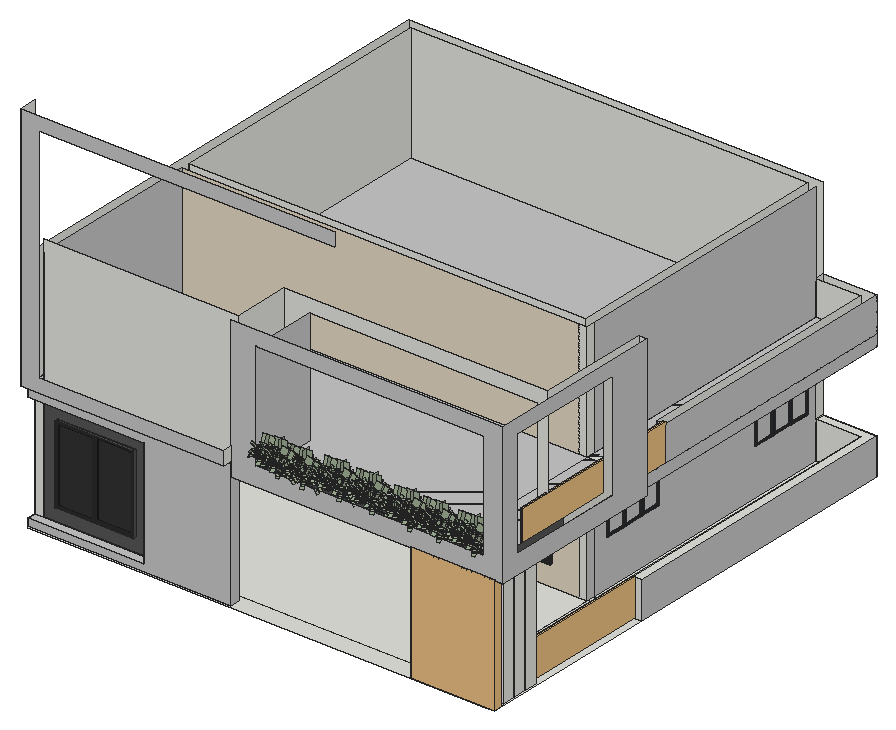
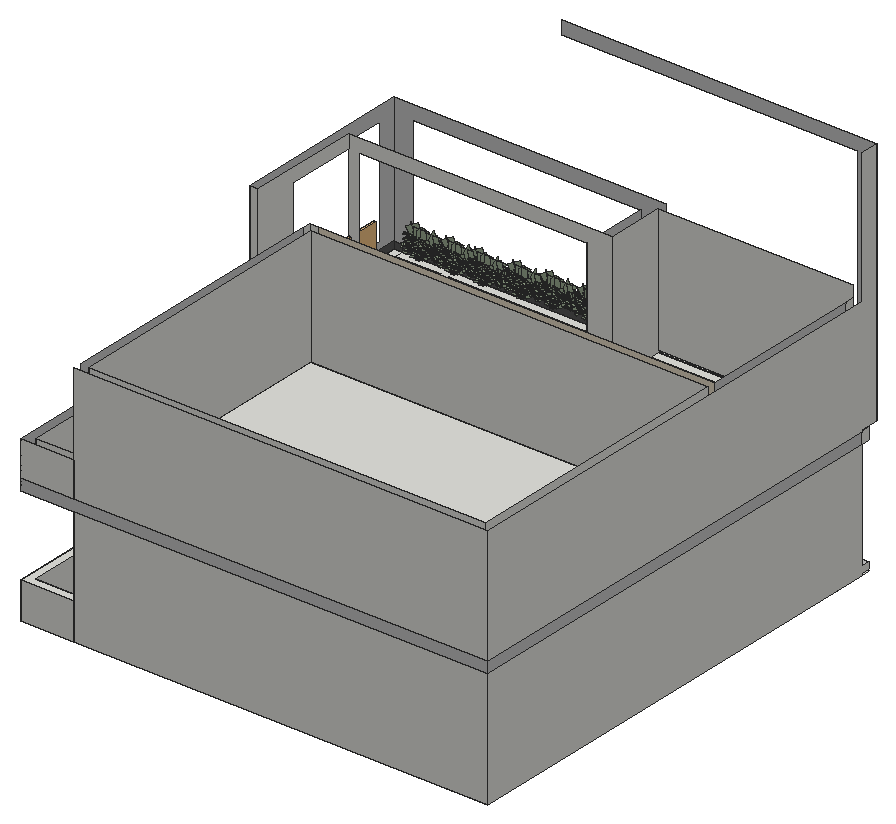
# SketchUp Ruby script. Lengths in inches.
U = 1.inch
M = Sketchup.active_model
def pt(a) = Geom::Point3d.new(a.map { |v| v * U })
def face(e, loops, mat)
  f = e.add_face(loops[0].map { |a| pt(a) })
  loops[1..].each { |l| e.add_face(l.map { |a| pt(a) }).erase! }
  f.material = f.back_material = mat if mat
  f
end
# faces: each face lists its corners as indices into pts; further lists are holes
def faces(e, pts, list, mat = nil) = list.each { |f| face(e, (f[0].is_a?(Array) ? f : [f]).map { |l| l.map { |i| pts[i] } }, mat) }
# xy, xz, yz: faces in a plane at the given z, y or x. An outline is a flat list of corners, or four numbers for a rectangle; further outlines are holes
def ring(l) = l.size == 4 ? [[l[0], l[1]], [l[2], l[1]], [l[2], l[3]], [l[0], l[3]]] : l.each_slice(2).to_a
def flat(e, list, mat, &to3) = list.each { |f| face(e, (f[0].is_a?(Array) ? f : [f]).map { |l| ring(l).map { |u, v| to3.(u, v) } }, mat) }
def xy(e, z, list, mat = nil) = flat(e, list, mat) { |x, y| [x, y, z] }
def xz(e, y, list, mat = nil) = flat(e, list, mat) { |x, z| [x, y, z] }
def yz(e, x, list, mat = nil) = flat(e, list, mat) { |y, z| [x, y, z] }
def lines(e, pts, list) = list.each { |a, b| e.add_line(pt(pts[a]), pt(pts[b])) }
# prism: a flat outline (further loops are holes) pulled along v
def prism(e, loops, v, mat = nil)
  f = face(e, loops, mat); d = Geom::Vector3d.new(v.map { |x| x * U })
  f.pushpull(f.normal.samedirection?(d) ? d.length : -d.length)
end
def box(e, o, s, mat = nil) = prism(e, [[o, [o[0] + s[0], o[1], o[2]], [o[0] + s[0], o[1] + s[1], o[2]], [o[0], o[1] + s[1], o[2]]]], [0, 0, s[2]], mat)
def at(x, y, z, deg = 0) = Geom::Transformation.translation(pt([x, y, z])) * Geom::Transformation.rotation(ORIGIN, Z_AXIS, deg.degrees)
def axes(o, x, y, z) = Geom::Transformation.new([*x, 0, *y, 0, *z, 0, *pt(o).to_a, 1])
def part(name) = M.definitions.add(name)
# library, detail: a bought-in or finely detailed component or shape, given as its bounding box
def library(name, o, s) = part(name).tap { |d| box(d.entities, o, s) }
def detail(e, o, s) = box(e.add_group.entities, o, s)
def put(e, d, t, mat = nil) = e.add_instance(d, t).tap { |i| i.material = mat if mat }
def group(e, t, mat = nil) = e.add_group.tap { |g| g.transformation = t; g.material = mat if mat }.entities
root = M.entities
M.materials.add("Glass_Tinted_Gray").color = [0, 0, 0]
M.materials["Glass_Tinted_Gray"].alpha = 0.125
M.materials.add("Wine2").color = [0, 0, 0]
M.materials["Wine2"].alpha = 0
M.materials.add("[0130_Gainsboro]").color = [39, 45, 50]
M.materials.add("[0135_DarkGray]").color = [81, 81, 81]
M.materials.add("[Color M02]").color = [198, 198, 198]
M.materials.add("[Color M06]").color = [86, 86, 86]
M.materials.add("[Mirror 02]").color = [229, 229, 229]
M.materials.add("[Stone Brushed Khaki]").color = [226, 216, 194]
M.materials.add("[Terrazzo Light Blue]").color = [196, 214, 227]
M.materials.add("hymenocallis littoralis").color = [156, 172, 146]
c1 = library("CNC CUTTING TEXTURE",[0,0,-0.79],[85.98,295.47,0.79])
c2 = part("Group\#3")
box(c2.entities,[0,0,0],[3.8125,11.9375,120])
c3 = library("Wagner Glass Railing",[9.08,102.375,1.53],[2.51,145.5,42.05])
c4 = part("Facade screen panel")
xy(c4.entities,0,[[0,-0.98,43.07,0],[0,0,43.07,1.4]],"[0130_Gainsboro]")
xy(c4.entities,0.3,[[0.3,-1.43,42.77,-0.98]],"[0130_Gainsboro]")
xy(c4.entities,2.95,[[2.95,-1.43,40.12,-0.63],[2.95,-0.63,40.12,0],[2.95,0,40.12,0.64],[2.95,0.64,40.12,1.4]],"[0130_Gainsboro]")
xy(c4.entities,3.54,[[3.54,-0.63,39.53,0],[3.54,0,39.53,0.64]],"[0130_Gainsboro]")
xy(c4.entities,111.8125,[[3.54,-0.63,39.53,0],[3.54,0,39.53,0.64]],"[0130_Gainsboro]")
xy(c4.entities,112.4,[[2.95,-1.43,40.12,-0.63],[2.95,-0.63,40.12,0],[2.95,0,40.12,0.64],[2.95,0.64,40.12,1.4]],"[0130_Gainsboro]")
xy(c4.entities,115.05,[[0.3,-1.43,42.77,-0.98]],"[0130_Gainsboro]")
xy(c4.entities,115.35,[[0,-0.98,43.07,0],[0,0,43.07,1.4]],"[0130_Gainsboro]")
xz(c4.entities,-1.43,[[[0.3,0.3,42.77,115.05],[2.95,2.95,40.12,112.4]]],"[0130_Gainsboro]")
xz(c4.entities,-0.98,[[[0,0,43.07,115.35],[0.3,0.3,42.77,115.05]]],"[0130_Gainsboro]")
xz(c4.entities,-0.63,[[[2.95,2.95,40.12,112.4],[3.54,3.54,39.53,111.8125]]],"[0130_Gainsboro]")
xz(c4.entities,0,[[3.54,3.54,39.53,111.8125]],"Wine2")
xz(c4.entities,0,[[[0,0,43.07,115.35],[2.95,2.95,40.12,112.4]],[[2.95,2.95,40.12,112.4],[3.54,3.54,39.53,111.8125]]],"[0130_Gainsboro]")
xz(c4.entities,0.64,[[[2.95,2.95,40.12,112.4],[3.54,3.54,39.53,111.8125]]],"[0130_Gainsboro]")
xz(c4.entities,1.4,[[[0,0,43.07,115.35],[2.95,2.95,40.12,112.4]]],"[0130_Gainsboro]")
yz(c4.entities,0,[[-0.98,0,0,115.35],[0,0,1.4,115.35]],"[0130_Gainsboro]")
yz(c4.entities,0.3,[[-1.43,0.3,-0.98,115.05]],"[0130_Gainsboro]")
yz(c4.entities,2.95,[[-1.43,2.95,-0.63,112.4],[-0.63,2.95,0,112.4],[0,2.95,0.64,112.4],[0.64,2.95,1.4,112.4]],"[0130_Gainsboro]")
yz(c4.entities,3.54,[[-0.63,3.54,0,111.8125],[0,3.54,0.64,111.8125]],"[0130_Gainsboro]")
yz(c4.entities,39.53,[[-0.63,3.54,0,111.8125],[0,3.54,0.64,111.8125]],"[0130_Gainsboro]")
yz(c4.entities,40.12,[[-1.43,2.95,-0.63,112.4],[-0.63,2.95,0,112.4],[0,2.95,0.64,112.4],[0.64,2.95,1.4,112.4]],"[0130_Gainsboro]")
yz(c4.entities,42.77,[[-1.43,0.3,-0.98,115.05]],"[0130_Gainsboro]")
yz(c4.entities,43.07,[[-0.98,0,0,115.35],[0,0,1.4,115.35]],"[0130_Gainsboro]")
c5 = part("Facade screen assembly")
put(c5.entities,c4,axes([90.57,1.43,0],[1.05148,0,0],[0,1,0],[0,0,1]))
put(c5.entities,c4,axes([0,1.43,0],[1.05148,0,0],[0,1,0],[0,0,1]))
put(c5.entities,c4,axes([45.29,1.43,0],[1.05148,0,0],[0,1,0],[0,0,1]))
c6 = part("PENTEK_RP Fineline 50S_Sliding_DoorCase_E1")
box(c6.entities,[0,0,0],[1.51,3.66,99.27],"[0135_DarkGray]")
c7 = part("PENTEK_RP Fineline 50S_SlidingDooe_Case_E2")
box(c7.entities,[0,0,0],[96.25,3.66,1.51],"[0135_DarkGray]")
c8 = part("pentek_RP Fineline 50S_SlidingDoor_Case")
put(c8.entities,c6,at(97.76,0,0))
put(c8.entities,c7,at(1.51,0,0))
put(c8.entities,c6,at(0,0,0))
put(c8.entities,c7,at(1.51,0,97.76))
c9 = part("PENTEK_RP Fineline 50S_SlidingDoor_GlazingBead_2")
box(c9.entities,[0,0,0],[0.56,0.59,94.39],"[0135_DarkGray]")
c10 = part("PENTEK_RP Fineline 50S_SlidingDoor_Glass")
box(c10.entities,[0,0,0],[46.58,0.16,94.39],"Glass_Tinted_Gray")
c11 = part("PENTEK_RP Fineline 50S_SlidingDoor_GlazingBead")
box(c11.entities,[0,0,0],[45.47,0.59,0.56],"[0135_DarkGray]")
c12 = part("PENTEK_RP Fineline 50S_SlidingDoor_Leaf_E1")
xy(c12.entities,0,[[0,0,0.93,1.97],[0.93,1.57,1.49,1.97]],"[0135_DarkGray]")
xy(c12.entities,96.25,[[0,0,0.93,0,0.93,1.57,1.49,1.57,1.49,1.97,0,1.97]],"[0135_DarkGray]")
xz(c12.entities,0,[[0,0,0.93,96.25]],"[0135_DarkGray]")
xz(c12.entities,1.57,[[0.93,0,1.49,95.32],[0.93,95.32,1.49,96.25]],"[0135_DarkGray]")
xz(c12.entities,1.97,[[0,0,1.49,96.25]],"[0135_DarkGray]")
yz(c12.entities,0,[[0,0,1.97,96.25]],"[0135_DarkGray]")
yz(c12.entities,0.93,[[0,0,1.57,0.93],[0,0.93,1.57,95.32],[0,95.32,1.57,96.25]],"[0135_DarkGray]")
yz(c12.entities,1.49,[[1.57,0,1.97,95.32],[1.57,95.32,1.97,96.25]],"[0135_DarkGray]")
c13 = part("PENTEK_RP Fineline 50S_SlidingDoor_Leaf_E2")
xy(c13.entities,0,[[0,0,0,1.57,0.56,1.57,0.56,1.97,46.02,1.97,46.02,1.57,46.58,1.57,46.58,0]],"[0135_DarkGray]")
xy(c13.entities,0.93,[[0,0,46.58,1.57]],"[0135_DarkGray]")
xy(c13.entities,1.49,[[0.56,1.57,46.02,1.97]],"[0135_DarkGray]")
xz(c13.entities,0,[[0,0,46.58,0.93]],"[0135_DarkGray]")
xz(c13.entities,1.57,[[0,0,0.56,0.93],[46.02,0,46.58,0.93],[0.56,0.93,46.02,1.49]],"[0135_DarkGray]")
xz(c13.entities,1.97,[[0.56,0,46.02,1.49]],"[0135_DarkGray]")
yz(c13.entities,0,[[0,0,1.57,0.93]],"[0135_DarkGray]")
yz(c13.entities,0.56,[[1.57,0,1.97,0.93],[1.57,0.93,1.97,1.49]],"[0135_DarkGray]")
yz(c13.entities,46.02,[[1.57,0,1.97,0.93],[1.57,0.93,1.97,1.49]],"[0135_DarkGray]")
yz(c13.entities,46.58,[[0,0,1.57,0.93]],"[0135_DarkGray]")
c14 = part("PENTEK_RP Fineline S_SlidingDoor_Leaf1")
put(c14.entities,c9,at(0.93,0,0.93))
put(c14.entities,c9,at(46.96,0,0.93))
put(c14.entities,c10,at(1.49,1.42,0.93))
put(c14.entities,c11,at(1.49,0,0.93))
put(c14.entities,c10,at(1.49,0.59,0.93),"[Terrazzo Light Blue]")
put(c14.entities,c12,at(0,0,0))
put(c14.entities,c12,axes([48.44,0,0],[-1,0,0],[0,1,0],[0,0,1]))
put(c14.entities,c13,axes([0.93,0,96.25],[1,0,0],[0,1,0],[0,0,-1]))
put(c14.entities,c13,at(0.93,0,0))
put(c14.entities,c11,at(1.49,0,94.77))
c15 = part("PENTEK_RP Fineline 50S_SlidingDoor_Leaf2")
put(c15.entities,c10,at(1.49,1.42,0.93))
put(c15.entities,c11,at(1.49,0,94.77))
put(c15.entities,c9,at(46.96,0,0.93))
put(c15.entities,c10,at(1.49,0.59,0.93),"[Mirror 02]")
put(c15.entities,c9,at(0.93,0,0.93))
put(c15.entities,c12,at(0,0,0))
put(c15.entities,c12,axes([48.44,0,0],[-1,0,0],[0,1,0],[0,0,1]))
put(c15.entities,c11,at(1.49,0,0.93))
put(c15.entities,c13,axes([0.93,0,96.25],[1,0,0],[0,1,0],[0,0,-1]))
put(c15.entities,c13,at(0.93,0,0))
c16 = part("PENTEK - Slimmest Steel Sliding Door / Window\#1")
put(c16.entities,c8,at(0,-1.88,-0.09))
put(c16.entities,c14,at(1.51,-2.27,1.42))
put(c16.entities,c15,at(49.32,-0.3,1.42))
c17 = part("Group\#1")
prism(c17.entities,[[[0,0,12],[425.4375,0,12],[480,0,12],[480,0,0],[0,0,0]]],[0,-480,0])
c18 = part("Group\#856")
xy(c18.entities,7.38,[[0,0,5.5,15.91]],"hymenocallis littoralis")
p = [[5.5,28.78,0],[5.5,26.79,3.44],[0,26.79,3.44],[0,28.78,0],[0,23.75,6],[5.5,23.75,6],
  [0,15.91,7.38],[5.5,15.91,7.38]]
faces(c18.entities,p,[[0,1,2,3],[4,2,1,5],[6,4,5,7]],"hymenocallis littoralis")
c19 = part("Group\#854")
xy(c19.entities,7.38,[[0,0,5.5,15.91],[0,15.91,5.5,23.87]],"hymenocallis littoralis")
p = [[5.5,31.07,4.3],[5.5,27.74,6.47],[0,27.74,6.47],[0,31.07,4.3],[0,23.87,7.38],[5.5,23.87,7.38]]
faces(c19.entities,p,[[0,1,2,3],[4,2,1,5]],"hymenocallis littoralis")
c20 = part("Group\#857")
xy(c20.entities,7.38,[[0,0,5.6,15.91]],"hymenocallis littoralis")
p = [[5.6,28.78,0],[5.6,26.79,3.44],[0,26.79,3.44],[0,28.78,0],[0,23.75,6],[5.6,23.75,6],
  [0,15.91,7.38],[5.6,15.91,7.38]]
faces(c20.entities,p,[[0,1,2,3],[4,2,1,5],[6,4,5,7]],"hymenocallis littoralis")
c21 = part("Group\#855")
put(c21.entities,c19,axes([6.09,8.57,-0.52],[0.446,0.85617,0.26089],[-0.18444,-0.19731,0.96283],[0.87582,-0.47754,0.0699]))
put(c21.entities,c19,axes([6.29,7.28,-1.71],[0.37058,0.92707,-0.05667],[-0.32382,0.19004,0.99128],[0.87712,-0.32925,0.34964]))
put(c21.entities,c19,axes([11.04,16.14,-0.7],[1,0,0],[0,0.16628,1.02662],[0,-1.18456,0.19186]))
c22 = part("Group\#860")
put(c22.entities,c18,axes([24.57,32.05,-1.76],[0.9552,-0.22102,-0.19681],[0.4036,0.95545,0.88585],[-0.00568,-0.67859,0.7345]))
put(c22.entities,c18,axes([23.95,29.24,-2.4],[0,1,0],[-0.76041,0,0.64945],[0.64945,0,0.76041]))
put(c22.entities,c18,axes([24.22,24.72,-0.48],[-0.70711,0.70711,0],[-0.32757,-0.32757,0.80237],[0.61237,0.61237,0.5]))
put(c22.entities,c19,axes([20.66,37.22,-0.63],[1.12361,0.03262,0.39091],[-0.43499,0.29739,0.78777],[0.09852,-1.27434,0.37535]))
put(c22.entities,c18,axes([28.75,24.45,-2.4],[-1,0,0],[0,-0.76041,0.64945],[0,0.64945,0.76041]))
put(c22.entities,c20,axes([30.4,30.98,-3.7],[0.65676,-0.72002,0.22414],[0.55667,0.66341,0.5],[-0.50871,-0.20361,0.83652]))
put(c22.entities,c20,axes([32.41,29.61,-3.7],[0.04029,-0.97372,0.22414],[0.85287,0.15038,0.5],[-0.52057,0.17102,0.83652]))
put(c22.entities,c18,axes([31.89,25.85,-1.76],[-0.92056,0.33739,-0.19681],[-0.5186,-0.89824,0.88585],[0.08952,0.67268,0.7345]))
put(c22.entities,c18,axes([25.55,34.78,-0.48],[0.86603,0.5,0],[-0.25,0.43301,0.86603],[0.43301,-0.75,0.5]))
put(c22.entities,c20,axes([20.4,16.9375,-8.07],[-0.70711,0.70711,0],[-0.35754,-0.35754,0.65422],[1.3987,1.3987,1.52882]))
put(c22.entities,c18,axes([32.86,34.14,-0.48],[0.76604,-0.64279,0],[0.32139,0.38302,0.86603],[-0.55667,-0.66341,0.5]))
put(c22.entities,c18,axes([27.15,34.7,-0.1],[0.82472,-0.17528,-0.53769],[0.53769,0.53769,0.64945],[0.17528,-0.82472,0.53769]))
put(c22.entities,c18,axes([33.58,28.77,-2.4],[0,-1,0],[0.76041,0,0.64945],[-0.64945,0,0.76041]))
put(c22.entities,c18,axes([26.43,23.87,-2.81],[-0.75126,0.04415,0.65853],[0.53769,-0.53769,0.64945],[0.38276,0.84199,0.3802]))
put(c22.entities,c18,axes([28.78,23.98,-2.4],[-1,0,0],[0,-0.76041,0.64945],[0,0.64945,0.76041]))
put(c22.entities,c18,axes([25.39,25.38,-2.4],[-0.70711,0.70711,0],[-0.53769,-0.53769,0.64945],[0.45923,0.45923,0.76041]))
put(c22.entities,c18,axes([27.32,21.63,-0.1],[-0.45923,0.70711,-0.53769],[-0.76041,0,0.64945],[0.45923,0.70711,0.53769]))
put(c22.entities,c18,axes([25.17,27.625,-1.76],[0.56416,0.80187,-0.19681],[-0.66673,0.66673,0.80532],[0.62659,-0.26057,0.7345]))
put(c22.entities,c20,axes([27.59,27.04,-3.96],[-0.8993,-0.06127,0.43301],[0.2962,-0.8138,0.5],[0.32175,0.57791,0.75]))
put(c22.entities,c20,axes([26.98,24.5,-3.18],[-0.5,0.86603,0],[-0.75,-0.43301,0.5],[0.43301,0.25,0.86603]))
put(c22.entities,c20,axes([24.55,27.74,-3.7],[0.29517,0.92878,0.22414],[-0.85287,0.15038,0.5],[0.43068,-0.33875,0.83652]))
put(c22.entities,c20,axes([24.26,29.8,-3.18],[0.76604,0.64279,0],[-0.47317,0.5639,0.425],[0.32139,-0.38302,0.86603]))
put(c22.entities,c20,axes([25.98,32.46,-3.18],[1,0,0],[0,0.86603,0.5],[0,-0.5,0.86603]))
put(c22.entities,c18,axes([28.78,33.57,-2.4],[1,0,0],[0,0.76041,0.64945],[0,-0.64945,0.76041]))
put(c22.entities,c21,at(14.99,21.38,2.5))
put(c22.entities,c19,axes([34.63,26.34,-1.46],[-0.70089,-0.70877,0.07994],[0.4756,-0.38088,0.79293],[-0.53156,0.59378,0.60405]))
put(c22.entities,c19,axes([28.14,16.92,1.8125],[-1.19719,0.6912,0],[-0.09607,-0.16641,0.94244],[0.68444,1.18549,0.17613]))
put(c22.entities,c19,axes([31.5625,35.84,0.97],[0.66765,-1.1564,0.35779],[0.04445,0.30732,0.91033],[-1.20828,-0.64496,0.17012]))
put(c22.entities,c19,axes([38.94,22.51,0.89],[-0.97932,-0.67164,-0.05202],[0.27787,-0.41401,0.90999],[-0.85985,0.93577,0.32097]))
put(c22.entities,c19,axes([38.44,21.09,1.98],[-1.02864,-0.54856,0.2395],[0.33481,0.06999,0.88388],[-0.77261,1.08328,0.06417]))
put(c22.entities,c20,axes([35.02,30.51,-1.3],[-0.17365,-0.98481,0],[0.60224,-0.10619,0.79122],[-0.7792,0.13739,0.61153]))
put(c22.entities,c20,axes([29.41,22.33,-1.3],[-0.93969,0.34202,0],[-0.20915,-0.57465,0.79122],[0.27061,0.74351,0.61153]))
put(c22.entities,c19,axes([19.64,36,-1.62],[1.18194,0.09546,0.08234],[-0.14377,0.68823,0.76313],[0.21457,-1.1326,0.62386]))
put(c22.entities,c20,axes([24.25,24.14,-1.3],[-0.34202,0.93969,0],[-0.57465,-0.20915,0.79122],[0.74351,0.27061,0.61153]))
put(c22.entities,c20,axes([25.98,34.61,-1.3],[1,0,0],[0,0.61153,0.79122],[0,-0.79122,0.61153]))
put(c22.entities,c20,axes([31.16,34.41,-1.64],[0.56518,-0.80224,-0.19234],[0.73413,0.34233,0.72935],[-0.47639,-0.50772,0.71782]))
put(c22.entities,c20,axes([40.52,26.84,-5.82],[-0.42262,-0.90631,0],[0.48019,-0.22391,0.68552],[-1.43418,0.66877,1.22305]))
put(c22.entities,c18,axes([29.86,38.42,-1.01],[0.89064,-0.37013,0.26413],[-0.03924,0.63286,1.01918],[-0.45353,-0.76487,0.45748]))
put(c22.entities,c18,axes([29.34,22.4,-0.48],[-0.99619,-0.08716,0],[0.04358,-0.4981,0.86603],[-0.07548,0.86273,0.5]))
c23 = part("Group\#858")
xz(c23.entities,10.07,[[9.07,0,10.07,31.01],[0,31.01,0,45.12,20.13,45.12,20.13,31.01,10.07,31.01,10.07,32.58,9.07,32.58,9.07,31.01]],"hymenocallis littoralis")
yz(c23.entities,10.07,[[0,31.01,20.13,45.12]],"hymenocallis littoralis")
p = [[9.57,9.2,0],[10.07,10.07,0],[10.07,10.07,31.01],[10.07,10.07,32.58],[9.57,9.2,32.58]]
faces(c23.entities,p,[[0,1,2,3,4]],"hymenocallis littoralis")
c24 = part("cây lá nắng")
put(c24.entities,c22,axes([49.26,-2.75,0],[0.63109,0.63109,0],[-0.63109,0.63109,0],[0,0,0.935]))
g1 = group(c24.entities,at(26.6,-8.68,0))
put(g1,c18,axes([-4.72,35.73,-1.65],[0.74231,0.46334,-0.18402],[-0.34827,0.85768,0.82827],[0.42467,-0.43184,0.68675]))
put(g1,c18,axes([-3.34,33.57,-2.24],[-0.63109,0.63109,0],[-0.47989,-0.47989,0.60723],[0.40986,0.40986,0.71098]))
put(g1,c18,axes([-0.3125,30.89,-0.45],[-0.8925,0,0],[0,-0.41345,0.75022],[0,0.77293,0.4675]))
put(g1,c19,axes([-10.79,39.66,-0.59],[0.68852,0.72969,0.3655],[-0.4622,-0.08684,0.73657],[0.86641,-0.74205,0.35095]))
put(g1,c18,axes([2.71,33.57,-2.24],[-0.63109,-0.63109,0],[0.47989,-0.47989,0.60723],[-0.40986,0.40986,0.71098]))
put(g1,c20,axes([-0.37,38.74,-3.46],[0.86887,-0.03992,0.20957],[-0.06737,0.76999,0.4675],[-0.19255,-0.44954,0.78214]))
put(g1,c20,axes([1.76,39.14,-3.46],[0.63993,-0.58908,0.20957],[0.44333,0.63315,0.4675],[-0.43646,-0.2206,0.78214]))
put(g1,c18,axes([3.81,36.4375,-1.65],[-0.79389,-0.36803,-0.18402],[0.23959,-0.89415,0.82827],[-0.36803,0.48102,0.68675]))
put(g1,c18,axes([-5.83,38.07,-0.45],[0.231,0.86209,0],[-0.43104,0.1155,0.80973],[0.74659,-0.20005,0.4675]))
put(g1,c20,axes([2.18,23.5625,-7.55],[-0.8925,0,0],[0,-0.45128,0.6117],[0,1.76542,1.42944]))
put(g1,c18,axes([-0.8125,42.28,-0.45],[0.8891,0.07779,0],[-0.03889,0.44455,0.80973],[0.06737,-0.76999,0.4675]))
put(g1,c18,axes([-4.76,39.03,-0.09],[0.63109,0.40986,-0.50274],[0,0.67866,0.60723],[0.63109,-0.40986,0.50274]))
put(g1,c18,axes([3.03,39.35,-2.24],[0.63109,-0.63109,0],[0.47989,0.47989,0.60723],[-0.40986,-0.40986,0.71098]))
put(g1,c18,axes([1.61,31.74,-2.625],[-0.50198,-0.44625,0.61573],[0.67866,0,0.60723],[-0.28982,0.77293,0.35549]))
put(g1,c18,axes([3.03,33.3,-2.24],[-0.63109,-0.63109,0],[0.47989,-0.47989,0.60723],[-0.40986,0.40986,0.71098]))
put(g1,c18,axes([0.01,32.04,-2.24],[-0.8925,0,0],[0,-0.67866,0.60723],[0,0.57963,0.71098]))
put(g1,c18,axes([3.59,30.89,-0.09],[-0.73607,0.15643,-0.50274],[-0.47989,-0.47989,0.60723],[-0.15643,0.73607,0.50274]))
put(g1,c18,axes([-1.55,33.32,-1.65],[-0.15002,0.86209,-0.18402],[-0.84154,0,0.75297],[0.55988,0.231,0.68675]))
put(g1,c20,axes([0.35,34.48,-3.71],[-0.52887,-0.60621,0.40487],[0.70051,-0.32665,0.4675],[-0.16166,0.56777,0.70125]))
put(g1,c20,axes([2.61,39.13,-1.74],[-0.86209,0.231,0],[-0.23031,-0.85954,0.15531],[0.03162,0.11799,0.91645]))
put(g1,c20,axes([-2.02,33,-3.46],[-0.39986,0.77243,0.20957],[-0.63315,-0.44333,0.4675],[0.48558,0.05802,0.78214]))
put(g1,c20,axes([-3.49,34.12,-2.97],[0.07779,0.8891,0],[-0.65449,0.05726,0.39737],[0.44455,-0.03889,0.80973]))
put(g1,c20,axes([-4.09,36.88,-2.97],[0.63109,0.63109,0],[-0.54654,0.54654,0.4675],[0.31555,-0.31555,0.80973]))
put(g1,c18,axes([-3.02,39.35,-2.24],[0.63109,0.63109,0],[-0.47989,0.47989,0.60723],[0.40986,-0.40986,0.71098]))
put(g1,c21,axes([-4.03,22.95,2.33],[0.63109,0.63109,0],[-0.63109,0.63109,0],[0,0,0.935]))
put(g1,c19,axes([5.24,38.48,-1.37],[0.00497,-0.88963,0.07474],[0.54052,0.05978,0.74139],[-0.71019,0.03927,0.56479]))
put(g1,c19,axes([7.08,28.4375,1.7],[-1.19175,-0.31933,0],[0.04439,-0.16565,0.88118],[-0.31621,1.1801,0.16468]))
put(g1,c19,axes([-2.7,42.54,0.91],[1.15114,-0.30845,0.33454],[-0.1659,0.22199,0.85115],[-0.3555,-1.16957,0.15907]))
put(g1,c19,axes([10.37,38.78,0.83],[-0.19417,-1.04191,-0.04864],[0.43664,-0.08592,0.85084],[-1.1332,0.04791,0.30011]))
put(g1,c19,axes([10.95,37.5625,1.85],[-0.30298,-0.99536,0.22393],[0.16713,0.25547,0.82643],[-1.17124,0.19607,0.06]))
put(g1,c20,axes([2.84,41.36,-1.22],[0.51192,-0.73109,0],[0.44708,0.31305,0.73979],[-0.57846,-0.40504,0.57178]))
put(g1,c20,axes([4.47,32.65,-1.22],[-0.80888,-0.37719,0],[0.23066,-0.49465,0.73979],[-0.29844,0.64,0.57178]))
put(g1,c19,axes([-10.32,35.12,-1.51],[0.68567,0.80616,0.07699],[-0.52507,0.3436,0.71352],[0.85019,-0.57936,0.58331]))
put(g1,c20,axes([0.07,30.54,-1.22],[-0.80888,0.37719,0],[-0.23066,-0.49465,0.73979],[0.29844,0.64,0.57178]))
put(g1,c20,axes([-5.45,38.24,-1.22],[0.63109,0.63109,0],[-0.38593,0.38593,0.73979],[0.49934,-0.49934,0.57178]))
put(g1,c20,axes([-2.05,41.38,-1.53],[0.86296,-0.14961,-0.17984],[0.24726,0.67935,0.68194],[0.01977,-0.62107,0.67116]))
put(g1,c20,axes([8.63,42.51,-5.4375],[0.30525,-0.83868,0],[0.44435,0.16173,0.64096],[-1.32716,-0.48305,1.14356]))
put(g1,c18,axes([-5.4,43.09,-0.94],[0.79566,0.32849,0.24696],[-0.42416,0.37462,0.95293],[0.19648,-0.76892,0.42774]))
put(g1,c18,axes([4.38,32.65,-0.45],[-0.57369,-0.68369,0],[0.34185,-0.28684,0.80973],[-0.5921,0.49683,0.4675]))
put(g1,c20,axes([-2,33.84,-0.15],[-0.24601,0.85793,0],[-0.85539,-0.24528,0.15531],[0.11742,0.03367,0.91645]))
put(g1,c20,axes([0.17,30.83,-4.47],[-0.24601,0.85793,0],[-0.85539,-0.24528,0.15531],[0.11742,0.03367,0.91645]))
put(g1,c20,axes([-1.97,32.18,-4.47],[0.58524,0.67383,0],[-0.67184,0.58351,0.15531],[0.09222,-0.0801,0.91645]))
put(g1,c20,axes([-2,34.71,-4.47],[0.88392,-0.12346,0],[0.12309,0.88131,0.15531],[-0.0169,-0.12098,0.91645]))
put(g1,c20,axes([0.11,36.12,-4.47],[0.37822,-0.8084,0],[0.80601,0.37711,0.15531],[-0.11064,-0.05177,0.91645]))
put(c24.entities,c23,axes([29.71,14.29,6.94],[0.425,0.73612,0],[-0.6771,0.39092,-0.33349],[-0.26859,0.15507,0.72712]))
put(c24.entities,c23,axes([42.0625,26.12,6.94],[0.85,0,0],[0,0.78185,-0.33349],[0,0.33349,0.78185]))
put(c24.entities,c22,axes([7.3125,23.0625,0],[0.8925,0,0],[0,0.8925,0],[0,0,0.935]))
put(c24.entities,c23,axes([24.4375,40.23,2.05],[0.85,0,0],[0,0.85,0],[0,0,0.85]))
c25 = part("Planting 101")
put(c25.entities,c24,axes([21.34,32.96,-4.59],[0,-0.71,0],[-0.71,0,0],[0,0,0.71]))
xy(root,132,[[352.1875,121.8125,823.1875,121.8125,823.1875,308.68,361.1875,308.68,361.1875,131.75,352.1875,131.75],[823.1875,121.8125,832.1875,131.75],[[352.1875,131.75,361.1875,131.75,361.1875,308.68,777.625,308.68,777.625,611.75,352.1875,611.75],[361.1875,317.68,768.625,602.75]],[823.1875,131.75,832.1875,310.29],[777.625,308.68,823.1875,317.68],
  [361.1875,317.68,768.625,602.75],[777.625,317.68,823.1875,602.75]])
xy(root,133.67,[[352.1875,121.8125,561,131.75]])
xy(root,140.5625,[[352.1875,121.8125,471.94,131.75]],"[Color M02]")
xy(root,170.01,[[823.1875,310.29,832.1875,310.29,832.1875,611.75,777.625,611.75,777.625,602.75,823.1875,602.75]])
xy(root,252,[[352.1875,121.8125,471.94,131.75],[561,121.8125,561,131.75,832.1875,131.75,832.1875,306.4375,840.86,306.4375,840.86,121.8125],[[352.1875,131.75,361.1875,131.75,361.1875,308.68,777.625,308.68,777.625,611.75,352.1875,611.75],[361.1875,317.68,768.625,602.75]]])
xy(root,264,[[352.1875,121.8125,561,131.75],[[352.1875,131.75,361.1875,131.75,361.1875,308.68,777.625,308.68,777.625,611.75,352.1875,611.75],[361.1875,317.68,768.625,602.75]],[361.1875,131.75,561,140.75],[561,131.75,587.02,190.625],[587.02,131.75,587.02,140.75,768.625,140.75,768.625,308.68,777.625,308.68,777.625,140.75,823.1875,140.75,823.1875,131.75],
  [823.1875,131.75,832.1875,340.9375],[361.1875,140.75,561,140.75,561,190.625,587.02,190.625,587.02,140.75,768.625,140.75,768.625,308.68,361.1875,308.68],[777.625,140.75,823.1875,308.68],[777.625,308.68,823.1875,317.68],[361.1875,317.68,768.625,602.75],
  [777.625,317.68,823.1875,602.75]])
xy(root,265.92,[[352.1875,112.8125,561,131.75]])
xz(root,112.8125,[[352.1875,265.92,561,265.92,561,280.08,371.42,280.08,371.42,507.32,674.9375,507.32,674.9375,521.25,352.1875,521.25]],"[Color M02]")
xz(root,121.8125,[[352.1875,133.67,561,133.67,561,264,352.1875,264,352.1875,252,471.94,252,471.94,140.5625,352.1875,140.5625],[[561,252,840.86,396],[587.02,271.125,821.46,381.625]]],"[Color M02]")
xz(root,131.75,[[352.1875,132,361.1875,133.67],[361.1875,133.67,361.1875,140.5625,471.94,140.5625,471.94,252,352.1875,252,352.1875,264,561,264,561,133.67],[352.1875,140.5625,361.1875,252],[561,252,832.1875,264],[352.1875,264,361.1875,265.92],
  [361.1875,265.92,561,396]])
xz(root,131.75,[[361.1875,140.5625,471.94,252],[587.02,264,823.1875,271.125],[823.1875,264,832.1875,271.125]],"[Color M06]")
xz(root,190.625,[[561,264,587.02,264,587.02,381.625,821.46,381.625,821.46,271.125,832.1875,271.125,832.1875,396,561,396]])
xz(root,306.4375,[[832.1875,252,840.86,264],[832.1875,264,840.86,396]])
xz(root,308.68,[[768.625,132,777.625,252],[768.625,264,777.625,384]])
xz(root,308.68,[[361.1875,132,768.625,252],[361.1875,264,768.625,384]],"[Stone Brushed Khaki]")
xz(root,310.29,[[823.1875,132,832.1875,170.01]])
xz(root,317.68,[[361.1875,132,768.625,252],[361.1875,264,768.625,384]])
xz(root,340.9375,[[823.1875,264,832.1875,299.4375]])
xz(root,602.75,[[361.1875,132,768.625,252],[777.625,132,823.1875,170.01],[361.1875,264,768.625,384],[777.625,264,823.1875,299.4375]])
xz(root,611.75,[[352.1875,132,777.625,252],[777.625,132,832.1875,170.01],[352.1875,264,777.625,384],[777.625,264,832.1875,299.4375]])
yz(root,352.1875,[[131.75,132,131.75,133.67,121.8125,133.67,121.8125,140.5625,131.75,140.5625,131.75,252,611.75,252,611.75,132],[121.8125,252,131.75,264],[131.75,264,131.75,265.92,112.8125,265.92,112.8125,521.25,131.75,521.25,131.75,384,611.75,384,611.75,264]])
yz(root,361.1875,[[131.75,132,140.75,252],[317.68,132,602.75,252],[131.75,264,140.75,384],[317.68,264,602.75,384]])
yz(root,361.1875,[[140.75,132,308.68,252],[140.75,264,308.68,384]],"[Color M02]")
yz(root,471.94,[[121.8125,140.5625,131.75,252]])
yz(root,561,[[121.8125,252,131.75,264],[121.8125,264,190.625,264,190.625,396,131.75,396,131.75,265.92,121.8125,265.92],[112.8125,265.92,121.8125,280.08]])
yz(root,561,[[121.8125,133.67,131.75,252]],"[Color M02]")
yz(root,587.02,[[131.75,264,131.75,271.125,121.8125,271.125,121.8125,381.625,190.625,381.625,190.625,264]],"[Color M02]")
yz(root,768.625,[[317.68,132,602.75,252],[317.68,264,602.75,384]])
yz(root,777.625,[[602.75,132,611.75,170.01],[602.75,170.01,611.75,252],[308.68,264,317.68,384],[602.75,264,611.75,299.4375]])
yz(root,777.625,[[308.68,132,317.68,252],[317.68,132,602.75,252],[317.68,264,602.75,384]],"[Color M02]")
yz(root,823.1875,[[310.29,132,602.75,170.01],[340.9375,264,602.75,299.4375]])
yz(root,832.1875,[[131.75,252,306.4375,264],[209.96,264,306.4375,264,306.4375,396,190.625,396,190.625,381.625,262.46,381.625,262.46,271.125,209.96,271.125]])
yz(root,832.1875,[[310.29,132,611.75,170.01],[340.9375,264,611.75,299.4375]],"[Color M02]")
yz(root,832.1875,[[131.75,264,209.96,271.125]],"[Color M06]")
yz(root,840.86,[[[121.8125,252,306.4375,396],[139.96,271.125,262.46,381.625]]],"[Color M02]")
p = [[361.1875,140.75,132],[768.625,140.75,132],[777.625,140.75,132],[777.625,308.68,132]]
lines(root,p,[[0,1],[2,3]])
put(root,c1,axes([746.2,129.17,132],[1,0,0],[0,0,0.4085],[0,9.34,0]))
put(root,c2,at(826.43,135.61,132))
put(root,c2,at(826.43,149.74,132))
put(root,c2,at(826.43,164.68,132))
put(root,c3,axes([813.97,9.18,131.37],[1,0,0],[0,1.21599,0],[0,0,0.897]))
put(root,c5,axes([643.8,306.64,153.21],[0.72,0,0],[0,0.72,0],[0,0,0.72]))
put(root,c16,axes([376.25,129.06,156.13],[0.81,0,0],[0,0.81,0],[0,0,0.81]),"[Color M06]")
put(root,c5,axes([778.33,334.1,179.6],[0,0.4896,0],[-0.4896,0,0],[0,0,0.4896]))
put(root,c5,axes([778.33,524.47,179.6],[0,0.4896,0],[-0.4896,0,0],[0,0,0.4896]))
put(root,c17,at(352.1875,611.75,252),"[Color M02]")
put(root,c25,axes([727.125,129.43,270.43],[0,-0.53939,0],[1,0,0],[0,0,1]))
put(root,c25,axes([756.8125,129.43,270.43],[0,-0.53939,0],[1,0,0],[0,0,1]))
put(root,c25,axes([792.75,129.43,270.43],[0,-0.53939,0],[1,0,0],[0,0,1]))
put(root,c25,axes([688.23,129.43,272.33],[0,-0.53939,0],[1,0,0],[0,0,1]))
put(root,c25,axes([619.78,125.78,272.82],[0,-0.53939,0],[1,0,0],[0,0,1]))
put(root,c25,axes([656.37,127.67,273.67],[0,-0.53939,0],[1,0,0],[0,0,1]))
put(root,c3,axes([820.59,29.92,262.625],[1,0,0],[0,1.25473,0],[0,0,0.897]))
put(root,c25,axes([599.73,119.04,278.22],[0,-0.53939,0],[1,0,0],[0,0,1]))
